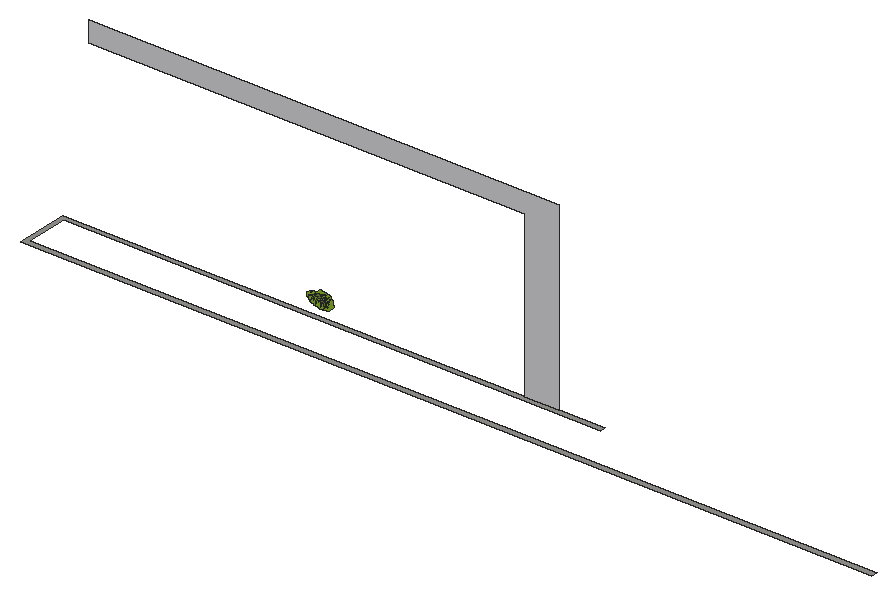
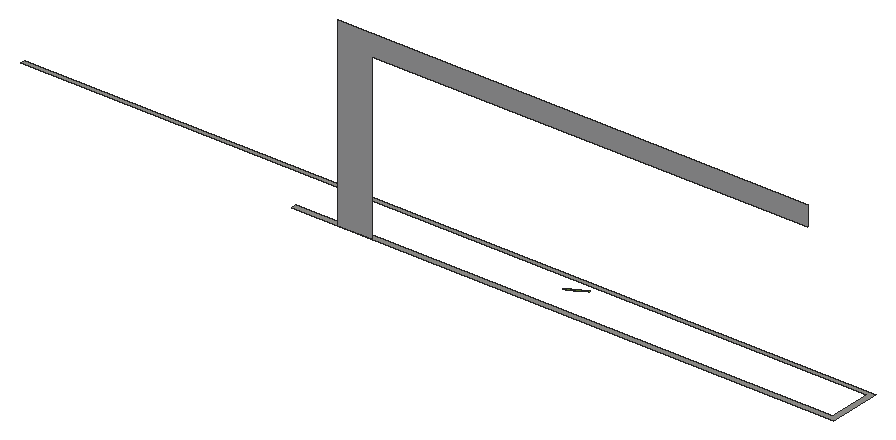
# SketchUp Ruby script. Lengths in inches.
U = 1.inch
M = Sketchup.active_model
def pt(a) = Geom::Point3d.new(a.map { |v| v * U })
def face(e, loops, mat)
  f = e.add_face(loops[0].map { |a| pt(a) })
  loops[1..].each { |l| e.add_face(l.map { |a| pt(a) }).erase! }
  f.material = f.back_material = mat if mat
  f
end
# faces: each face lists its corners as indices into pts; further lists are holes
def faces(e, pts, list, mat = nil) = list.each { |f| face(e, (f[0].is_a?(Array) ? f : [f]).map { |l| l.map { |i| pts[i] } }, mat) }
# xy, xz, yz: faces in a plane at the given z, y or x. An outline is a flat list of corners, or four numbers for a rectangle; further outlines are holes
def ring(l) = l.size == 4 ? [[l[0], l[1]], [l[2], l[1]], [l[2], l[3]], [l[0], l[3]]] : l.each_slice(2).to_a
def flat(e, list, mat, &to3) = list.each { |f| face(e, (f[0].is_a?(Array) ? f : [f]).map { |l| ring(l).map { |u, v| to3.(u, v) } }, mat) }
def xy(e, z, list, mat = nil) = flat(e, list, mat) { |x, y| [x, y, z] }
def xz(e, y, list, mat = nil) = flat(e, list, mat) { |x, z| [x, y, z] }
def yz(e, x, list, mat = nil) = flat(e, list, mat) { |y, z| [x, y, z] }
def lines(e, pts, list) = list.each { |a, b| e.add_line(pt(pts[a]), pt(pts[b])) }
# prism: a flat outline (further loops are holes) pulled along v
def prism(e, loops, v, mat = nil)
  f = face(e, loops, mat); d = Geom::Vector3d.new(v.map { |x| x * U })
  f.pushpull(f.normal.samedirection?(d) ? d.length : -d.length)
end
def box(e, o, s, mat = nil) = prism(e, [[o, [o[0] + s[0], o[1], o[2]], [o[0] + s[0], o[1] + s[1], o[2]], [o[0], o[1] + s[1], o[2]]]], [0, 0, s[2]], mat)
def at(x, y, z, deg = 0) = Geom::Transformation.translation(pt([x, y, z])) * Geom::Transformation.rotation(ORIGIN, Z_AXIS, deg.degrees)
def axes(o, x, y, z) = Geom::Transformation.new([*x, 0, *y, 0, *z, 0, *pt(o).to_a, 1])
def part(name) = M.definitions.add(name)
# library, detail: a bought-in or finely detailed component or shape, given as its bounding box
def library(name, o, s) = part(name).tap { |d| box(d.entities, o, s) }
def detail(e, o, s) = box(e.add_group.entities, o, s)
def put(e, d, t, mat = nil) = e.add_instance(d, t).tap { |i| i.material = mat if mat }
def group(e, t, mat = nil) = e.add_group.tap { |g| g.transformation = t; g.material = mat if mat }.entities
root = M.entities
M.materials.add("[0059_DarkOliveGreen]").color = [85, 107, 47]
M.materials.add("[0061_OliveDrab]").color = [107, 142, 35]
M.materials.add("[Granite Light Gray]").color = [149, 148, 144]
M.materials.add("[Polished Concrete New]").color = [200, 200, 203]
xy(root,7.8125,[[0,114.25,641.18,114.25,641.18,118.08,3.82,118.08,3.82,150.16,408.3,150.16,408.3,153.99,0,153.99]],"[Granite Light Gray]")
xz(root,153.99,[[347.76,7.8125,373.77,7.8125,373.77,146.4375,20.0625,146.4375,20.0625,131.1875,347.76,131.1875]],"[Polished Concrete New]")
p = [[199.93,152.92,25.19],[201.18,153.19,24.99],[202.33,153.03,24.625],[202.98,152.74,24.33],[203.54,152.19,23.94],[203.8,152.02,23.79],
  [202.43,151.98,24.13],[201.02,151.73,24.38],[199.67,151.35,24.56],[198.69,150.87,24.6],[198.51,150.72,24.58],[198.58,150.67,24.53],
  [198.92,150.73,24.48],[200.51,151.22,24.28],[201.92,151.53,24.0625],[203.44,151.8,23.79],[204.25,151.875,23.61],[204.95,151.76,23.38],
  [205.33,151.49,23.16],[205.74,151.04,22.86],[206.08,150.63,22.58],[206.25,150.42,22.45],[206.88,150.0625,22.125],[207.32,149.66,21.83],
  [207.59,149.24,21.57],[207.77,149.02,21.43],[207,149.06,21.64],[205.85,149.1,21.96],[207.91,148.68,21.24],[208.16,148.56,21.12],
  [208.23,148.18,20.93],[208.3,147.79,20.74],[207.77,146.91,20.48],[207.51,145.66,19.99],[206.23,145.15,20.09],[205.34,144.65,20.09],
  [204.84,144.32,20.08],[203.53,144.95,20.69],[202.82,145.44,21.1],[202.32,146.15,21.54],[202.01,146.65,21.85],[201.66,146.89,22.04],
  [201.375,147.09,22.21],[201.18,147.09,22.26],[201.12,146.96,22.21],[201.27,146.5625,22],[201.52,146.23,21.79],[202.32,145.54,21.27],
  [203.04,144.97,20.83],[203.44,144.61,20.5625],[203.91,144.37,20.34],[204.4,144.19,20.13],[203.63,143.93,20.21],[202.97,143.8125,20.33],
  [202.38,143.75,20.45],[201.91,143.72,20.56],[201.36,143.65,20.67],[200.34,144.22,21.18],[199.8,144.75,21.5625],[199.55,145.22,21.84],
  [199.27,146.09,22.3],[199.18,146.76,22.625],[199.0625,147.32,22.91],[198.9,147.74,23.14],[198.61,147.94,23.3],[198.22,147.95,23.41],
  [198.05,147.64,23.31],[197.95,147.21,23.14],[198.14,146.45,22.75],[198.64,145.64,22.26],[199.41,144.74,21.66],[200.6,143.72,20.9],
  [198.62,143.61,21.36],[197.44,143.59,21.65],[196.93,143.75,21.85],[196.39,144.125,22.16],[196.08,144.58,22.44],[195.96,145.19,22.75],
  [195.87,145.72,23.01],[195.77,146.49,23.38],[195.84,147.06,23.62],[195.89,147.5,23.8],[195.97,147.72,23.88],[195.79,147.85,23.99],
  [195.51,147.71,24],[195.17,147.38,23.9375],[195,146.87,23.75],[195.14,145.82,23.24],[195.36,145.2,22.91],[195.65,144.65,22.59],
  [195.93,144.4,22.4],[196.39,143.89,22.06],[196.0625,143.875,22.13],[194.92,144,22.48],[193.91,144.13,22.8],[192.75,144.64,23.33],
  [192.54,145.18,23.625],[192.7,146.03,23.97],[193.18,146.78,24.18],[193.53,147.47,24.4],[193.71,147.77,24.49],[193.67,147.94,24.57],
  [193.47,147.92,24.62],[193.04,147.57,24.57],[192.4375,146.73,24.35],[192.26,146.05,24.09],[192.27,144.96,23.6],[190.9,145.51,24.19],
  [190.18,146.0625,24.625],[190.06,146.53,24.87],[190.29,146.77,24.91],[191.05,147.49,25.04],[191.75,148.02,25.1],[192.1875,148.44,25.18],
  [192.24,148.61,25.24],[192.05,148.66,25.3125],[191.86,148.57,25.32],[190.94,147.9,25.26],[190.42,147.36,25.15],[190.07,146.875,25.02],
  [189.84,146.51,24.92],[189.34,146.96,25.25],[189.1875,147.38,25.47],[189.4,147.92,25.66],[189.85,148.43,25.78],[190.15,148.95,25.93],
  [190.71,149.22,25.91],[191.38,149.66,25.94],[192.17,150.05,25.9],[193.21,150.23,25.72],[194.3,150.17,25.41],[194.93,150.04,25.19],
  [195.16,150.3,25.25],[194.64,150.52,25.48],[194.11,150.89,25.78],[194.14,151.37,25.99],[194.54,152.07,26.2],[194.9375,152.71,26.39],
  [195.11,153.16,26.55],[197.39,153.43,26.08],[198.75,153.42,25.72],[199.55,153.1875,25.41],[203.37,151.12,23.5],[200.41,150.79,24.12],
  [198.45,150.23,24.37],[196.78,149.61,24.52],[196.3,149.78,24.72],[196.96,150.4,24.83],[197.84,151.23,24.97],[199.84,152.06,24.83],
  [198.04,151.49,25.04],[196.71,150.84,25.09],[196.1875,150.1,24.9],[195.94,149.99,24.91],[195.59,150.23,25.1],[196.29,151.39,25.45],
  [196.6,152.7,25.95],[195.23,150.09,25.14],[194.43,149.875,25.25],[192.7,149.53,25.54],[191.625,149.09,25.61],[191,148.7,25.6],
  [192.81,149.3,25.41],[194.3,149.65,25.18],[195.14,149.76,25.01],[193.8,149.27,25.13],[192.54,148.3,25.02],[191.875,147.52,24.84],
  [191.36,146.71,24.62],[191.2,146.31,24.48],[192.24,147.55,24.77],[192.98,148.29,24.91],[193.98,149.1,25.01],[194.85,149.52,24.98],
  [195.34,149.7,24.93],[195.64,149.66,24.84],[195.71,149.52,24.76],[195.41,149.16,24.67],[194.94,148.8,24.63],[194.63,148.375,24.52],
  [194.03,147.14,24.12],[193.84,146.35,23.8125],[194.02,145.61,23.4375],[194.13,145.01,23.14],[194.46,144.78,22.95],[194.22,145.94,23.53],
  [194.3,146.59,23.81],[194.64,147.625,24.18],[195.2,148.54,24.45],[195.98,149.54,24.69],[197.21,149.02,24.14],[196.92,148.25,23.875],
  [196.67,147.52,23.61],[196.91,146.01,22.875],[197.34,145.27,22.43],[197.71,144.77,22.11],[198.05,144.54,21.92],[197.65,145.24,22.34],
  [197.29,146.4,22.95],[197.17,147.89,23.65],[197.55,148.78,23.95],[199.9,147.99,22.99],[199.72,147.39,22.77],[199.96,146.65,22.375],
  [200.48,145.95,21.93],[201.04,145.42,21.54],[201.88,144.84,21.07],[200.69,146.04,21.91],[200.21,146.74,22.35],[200.05,147.39,22.68],
  [200.17,147.98,22.92],[202.01,147.47,22.22],[202.34,146.83,21.84],[202.91,146.25,21.4375],[203.59,145.78,21.05],[204.26,145.57,20.78],
  [203.11,146.36,21.43],[202.66,146.95,21.82],[202.39,147.43,22.1],[203.8125,146.94,21.51],[204.58,146.68,21.2],[205.55,146.31,20.79],
  [205.42,146.38,20.85],[203.99,147.09,21.54],[202.53,147.66,22.17],[200.79,148.09,22.81],[204.9,148.375,21.88],[200.22,148.375,23.08],
  [198.82,148.88,23.67],[200.83,149.34,23.36],[204.09,149.8125,22.73],[201.69,149.64,23.27],[199.48,149.3,23.6875],[198.31,149.02,23.86],
  [197.14,149.51,24.39],[199.67,150.32,24.1],[201.49,150.32,23.63],[200.13,150.05,23.85],[199.8,149.9,23.875],[199.72,149.8,23.85],
  [199.875,149.76,23.79],[200.42,149.84,23.6875],[201.72,150.04,23.45],[203.15,150.26,23.17],[204.65,150.42,22.86],[205.36,150.51,22.72],
  [203.22,150.49,23.26],[201.33,149.04,23.1],[200.84,148.91,23.16],[200.8125,148.76,23.1],[201.03,148.68,23.01],[201.51,148.66,22.88],
  [201.88,148.72,22.81],[203.39,148.91,22.51],[204.79,149.1,22.23],[202.65,149.12,22.79],[198.5625,152.52,25.37],[197.91,152.29,25.43],
  [197.3125,151.92,25.42],[196.97,151.6,25.36],[197,151.42,25.28],[197.16,151.37,25.21],[198.18,151.91,25.19],[198.99,152.39,25.2],
  [199.14,152.53,25.22],[196.25,148.42,24.125],[196.53,148.68,24.17],[196.46,149.01,24.33],[196.16,149.11,24.46],[195.87,148.89,24.43],
  [195.8125,148.61,24.32],[195.99,148.4,24.18],[194.86,149.37,24.91],[194.65,149.08,24.83],[194.64,148.87,24.74],[194.9,148.875,24.68],
  [195.12,149.1875,24.76],[195.14,149.42,24.86]]
faces(root,p,[[[0,1,2,3,4,5,6,7,8,9,10,11,12,13,14,15,16,17,18,19,20,21,22,23,24,25,26,27,28,29,30,31,32,33,34,35,36,37,38,39,40,41,42,43,44,45,46,47,48,49,50,51,52,53,54,55,56,57,58,59,60,61,62,63,64,65,66,67,68,69,70,71,72,73,74,75,76,77,78,79,80,81,82,83,84,85,86,87,88,89,90,75,91,92,93,94,95,96,97,98,99,100,101,102,103,104,105,106,107,108,109,110,111,112,113,114,115,116,117,118,119,120,121,122,123,124,125,126,127,128,129,130,131,132,133,134,135,136,137,138,139,140,141],[142,143,144,145,146,147,148,149,150,151,152,153,154,155,156,157,158,159,160,161,162,163,164,165,166,167,168,169,170,171,172,173,174,175,176,177,178,179,180,181,182,183,184,185,186,187,188,189,190,191,192,193,194,195,196,197,198,199,200,201,202,203,204,205,206,207,208,209,210,211,212,213,214,215,216,217,218,219,220,221,222,223,224,225,226,227,228,229,230,231,232,233,234,235],[236,237,238,239,240,241,242,243,244,245,246],[247,248,249,250,251,252,253,254,255],[256,257,258,259,260,261,262,263,264],[265,266,267,268,269,270,271],[272,273,274,275,276,277]]],"[0061_OliveDrab]")
faces(root,p,[[143,142,235,234,233,232,231,230,229,228,227,226,225,224,223,222,221,220,219,218,217,216,215,214,213,212,211,210,209,208,207,206,205,204,203,202,201,200,199,198,197,196,195,194,193,192,191,190,189,188,187,186,185,184,183,182,181,180,179,178,177,176,175,174,173,172,171,170,169,168,167,166,165,164,163,162,161,160,159,158,157,156,155,154,153,152,151,150,149,148,147,146,145,144]],"[0059_DarkOliveGreen]")
